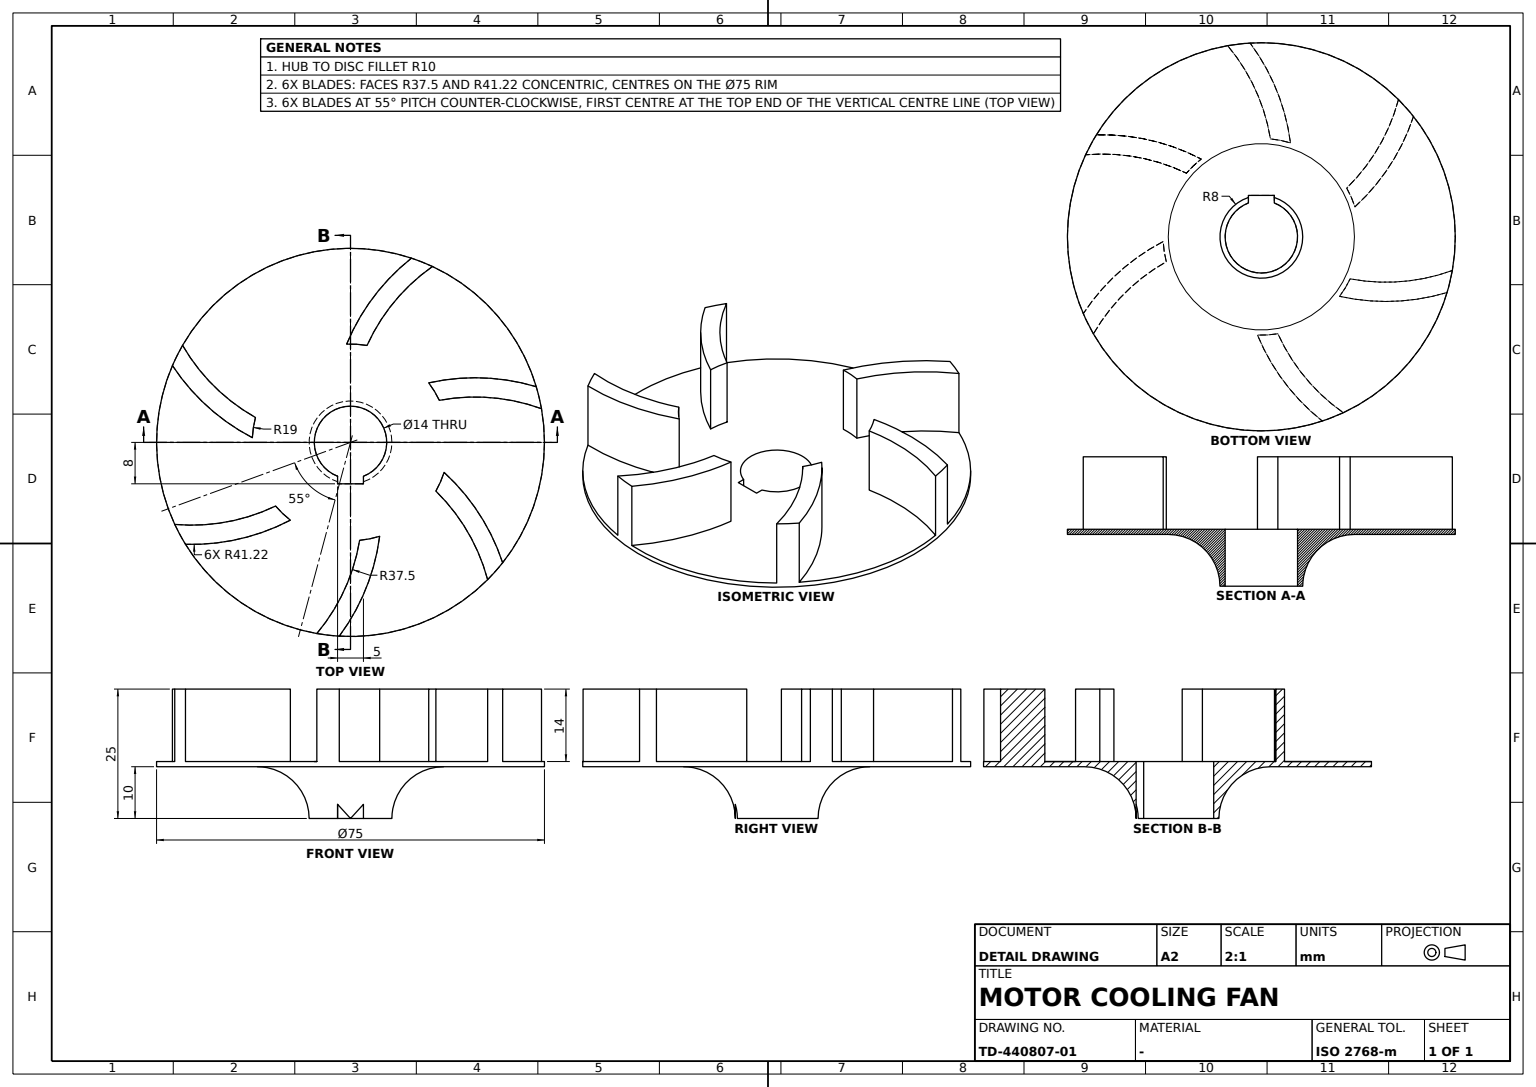
ISO-10303-21;
HEADER;
FILE_DESCRIPTION((''),'2;1');
FILE_NAME('','',(''),(''),'','','');
FILE_SCHEMA(('AUTOMOTIVE_DESIGN'));
ENDSEC;
DATA;
#1=APPLICATION_CONTEXT('');
#2=PRODUCT_CONTEXT('',#1,'mechanical');
#3=PRODUCT('','','',(#2));
#4=PRODUCT_DEFINITION_FORMATION('','',#3);
#5=PRODUCT_DEFINITION_CONTEXT('',#1,'design');
#6=PRODUCT_DEFINITION('','',#4,#5);
#7=PRODUCT_DEFINITION_SHAPE('','',#6);
#8=(LENGTH_UNIT()NAMED_UNIT(*)SI_UNIT(.MILLI.,.METRE.));
#9=(NAMED_UNIT(*)PLANE_ANGLE_UNIT()SI_UNIT($,.RADIAN.));
#10=(NAMED_UNIT(*)SI_UNIT($,.STERADIAN.)SOLID_ANGLE_UNIT());
#11=UNCERTAINTY_MEASURE_WITH_UNIT(LENGTH_MEASURE(0.005),#8,'distance_accuracy_value','');
#12=(GEOMETRIC_REPRESENTATION_CONTEXT(3)GLOBAL_UNCERTAINTY_ASSIGNED_CONTEXT((#11))GLOBAL_UNIT_ASSIGNED_CONTEXT((#8,#9,#10))REPRESENTATION_CONTEXT('',''));
#13=CARTESIAN_POINT('',(5.636932,-18.144558,1.));
#14=VERTEX_POINT('',#13);
#15=CARTESIAN_POINT('',(5.636932,-18.144558,15.));
#16=VERTEX_POINT('',#15);
#17=DIRECTION('',(0.,0.,1.));
#18=VECTOR('',#17,1000.);
#19=LINE('',#13,#18);
#20=EDGE_CURVE('',#14,#16,#19,.T.);
#21=ORIENTED_EDGE('',*,*,#20,.T.);
#22=CARTESIAN_POINT('',(-2.172274,-37.43703,15.));
#23=VERTEX_POINT('',#22);
#24=CARTESIAN_POINT('',(-35.238473,-12.825755,15.));
#25=DIRECTION('',(1.,0.,0.));
#26=AXIS2_PLACEMENT_3D('',#24,#17,#25);
#27=CIRCLE('',#26,41.22);
#28=EDGE_CURVE('',#23,#16,#27,.T.);
#29=ORIENTED_EDGE('',*,*,#28,.F.);
#30=CARTESIAN_POINT('',(-2.172274,-37.43703,1.));
#31=VERTEX_POINT('',#30);
#32=LINE('',#30,#18);
#33=EDGE_CURVE('',#31,#23,#32,.T.);
#34=ORIENTED_EDGE('',*,*,#33,.F.);
#35=CARTESIAN_POINT('',(-35.238473,-12.825755,1.));
#36=AXIS2_PLACEMENT_3D('',#35,#17,#25);
#37=CIRCLE('',#36,41.22);
#38=EDGE_CURVE('',#31,#14,#37,.T.);
#39=ORIENTED_EDGE('',*,*,#38,.T.);
#40=EDGE_LOOP('',(#21,#29,#34,#39));
#41=FACE_BOUND('',#40,.T.);
#42=CARTESIAN_POINT('',(-35.238473,-12.825755,8.));
#43=DIRECTION('',(-0.342020143,0.939692621,0.));
#44=AXIS2_PLACEMENT_3D('',#42,#17,#43);
#45=CYLINDRICAL_SURFACE('',#44,41.22);
#46=ADVANCED_FACE('',(#41),#45,.T.);
#47=CARTESIAN_POINT('',(2.5,-6.538348,1.));
#48=VERTEX_POINT('',#47);
#49=CARTESIAN_POINT('',(2.5,-8.,1.));
#50=VERTEX_POINT('',#49);
#51=CARTESIAN_POINT('',(2.5,0.,1.));
#52=DIRECTION('',(0.,-1.,0.));
#53=VECTOR('',#52,1000.);
#54=LINE('',#51,#53);
#55=EDGE_CURVE('',#48,#50,#54,.T.);
#56=ORIENTED_EDGE('',*,*,#55,.F.);
#57=CARTESIAN_POINT('',(2.5,-6.538348,-10.));
#58=VERTEX_POINT('',#57);
#59=DIRECTION('',(0.,0.,-1.));
#60=VECTOR('',#59,1000.);
#61=LINE('',#57,#60);
#62=EDGE_CURVE('',#58,#48,#61,.F.);
#63=ORIENTED_EDGE('',*,*,#62,.F.);
#64=CARTESIAN_POINT('',(2.5,-7.599342,-10.));
#65=VERTEX_POINT('',#64);
#66=LINE('',#57,#53);
#67=EDGE_CURVE('',#58,#65,#66,.T.);
#68=ORIENTED_EDGE('',*,*,#67,.T.);
#69=CARTESIAN_POINT('',(2.5,-8.,-7.264131));
#70=VERTEX_POINT('',#69);
#71=CARTESIAN_POINT('',(2.5,-7.734013,-8.156693));
#72=CARTESIAN_POINT('',(2.5,-7.599342,-9.068485));
#73=B_SPLINE_CURVE_WITH_KNOTS('',3,(#69,#71,#72,#64),.UNSPECIFIED.,.F.,.F.,(4,4),(0.,0.002765051),.UNSPECIFIED.);
#74=EDGE_CURVE('',#70,#65,#73,.T.);
#75=ORIENTED_EDGE('',*,*,#74,.F.);
#76=CARTESIAN_POINT('',(2.5,-8.,-10.));
#77=LINE('',#76,#60);
#78=EDGE_CURVE('',#50,#70,#77,.T.);
#79=ORIENTED_EDGE('',*,*,#78,.F.);
#80=EDGE_LOOP('',(#56,#63,#68,#75,#79));
#81=FACE_BOUND('',#80,.T.);
#82=DIRECTION('',(-1.,0.,0.));
#83=AXIS2_PLACEMENT_3D('',#57,#82,#52);
#84=PLANE('',#83);
#85=ADVANCED_FACE('',(#81),#84,.T.);
#86=CARTESIAN_POINT('',(3.193077,18.729769,1.));
#87=VERTEX_POINT('',#86);
#88=CARTESIAN_POINT('',(3.193077,18.729769,15.));
#89=VERTEX_POINT('',#88);
#90=LINE('',#86,#18);
#91=EDGE_CURVE('',#87,#89,#90,.T.);
#92=ORIENTED_EDGE('',*,*,#91,.F.);
#93=CARTESIAN_POINT('',(15.848185,33.986542,1.));
#94=VERTEX_POINT('',#93);
#95=CARTESIAN_POINT('',(37.357301,3.26834,1.));
#96=AXIS2_PLACEMENT_3D('',#95,#17,#25);
#97=CIRCLE('',#96,37.5);
#98=EDGE_CURVE('',#94,#87,#97,.T.);
#99=ORIENTED_EDGE('',*,*,#98,.F.);
#100=CARTESIAN_POINT('',(15.848185,33.986542,15.));
#101=VERTEX_POINT('',#100);
#102=LINE('',#93,#18);
#103=EDGE_CURVE('',#94,#101,#102,.T.);
#104=ORIENTED_EDGE('',*,*,#103,.T.);
#105=CARTESIAN_POINT('',(37.357301,3.26834,15.));
#106=AXIS2_PLACEMENT_3D('',#105,#17,#25);
#107=CIRCLE('',#106,37.5);
#108=EDGE_CURVE('',#101,#89,#107,.T.);
#109=ORIENTED_EDGE('',*,*,#108,.T.);
#110=EDGE_LOOP('',(#92,#99,#104,#109));
#111=FACE_BOUND('',#110,.T.);
#112=CARTESIAN_POINT('',(37.357301,3.26834,8.));
#113=DIRECTION('',(0.087155743,-0.996194698,0.));
#114=AXIS2_PLACEMENT_3D('',#112,#17,#113);
#115=CYLINDRICAL_SURFACE('',#114,37.5);
#116=ADVANCED_FACE('',(#111),#115,.F.);
#117=CARTESIAN_POINT('',(-32.475953,18.75,1.));
#118=VERTEX_POINT('',#117);
#119=CARTESIAN_POINT('',(-32.475953,18.75,15.));
#120=VERTEX_POINT('',#119);
#121=LINE('',#117,#18);
#122=EDGE_CURVE('',#118,#120,#121,.T.);
#123=ORIENTED_EDGE('',*,*,#122,.T.);
#124=CARTESIAN_POINT('',(-18.380202,4.813333,15.));
#125=VERTEX_POINT('',#124);
#126=CARTESIAN_POINT('',(0.,37.5,15.));
#127=AXIS2_PLACEMENT_3D('',#126,#17,#25);
#128=CIRCLE('',#127,37.5);
#129=EDGE_CURVE('',#120,#125,#128,.T.);
#130=ORIENTED_EDGE('',*,*,#129,.T.);
#131=CARTESIAN_POINT('',(-18.380202,4.813333,1.));
#132=VERTEX_POINT('',#131);
#133=LINE('',#131,#18);
#134=EDGE_CURVE('',#132,#125,#133,.T.);
#135=ORIENTED_EDGE('',*,*,#134,.F.);
#136=CARTESIAN_POINT('',(0.,37.5,1.));
#137=AXIS2_PLACEMENT_3D('',#136,#17,#25);
#138=CIRCLE('',#137,37.5);
#139=EDGE_CURVE('',#118,#132,#138,.T.);
#140=ORIENTED_EDGE('',*,*,#139,.F.);
#141=EDGE_LOOP('',(#123,#130,#135,#140));
#142=FACE_BOUND('',#141,.T.);
#143=CARTESIAN_POINT('',(0.,37.5,8.));
#144=AXIS2_PLACEMENT_3D('',#143,#17,#25);
#145=CYLINDRICAL_SURFACE('',#144,37.5);
#146=ADVANCED_FACE('',(#142),#145,.F.);
#147=ORIENTED_EDGE('',*,*,#67,.F.);
#148=CARTESIAN_POINT('',(-2.5,-6.538348,-10.));
#149=VERTEX_POINT('',#148);
#150=CARTESIAN_POINT('',(0.,0.,-10.));
#151=AXIS2_PLACEMENT_3D('',#150,#59,#82);
#152=CIRCLE('',#151,7.);
#153=EDGE_CURVE('',#149,#58,#152,.T.);
#154=ORIENTED_EDGE('',*,*,#153,.F.);
#155=CARTESIAN_POINT('',(-2.5,-7.599342,-10.));
#156=VERTEX_POINT('',#155);
#157=LINE('',#148,#53);
#158=EDGE_CURVE('',#149,#156,#157,.T.);
#159=ORIENTED_EDGE('',*,*,#158,.T.);
#160=AXIS2_PLACEMENT_3D('',#150,#17,#25);
#161=CIRCLE('',#160,8.);
#162=EDGE_CURVE('',#156,#65,#161,.F.);
#163=ORIENTED_EDGE('',*,*,#162,.T.);
#164=EDGE_LOOP('',(#147,#154,#159,#163));
#165=FACE_BOUND('',#164,.T.);
#166=AXIS2_PLACEMENT_3D('',#150,#59,#25);
#167=PLANE('',#166);
#168=ADVANCED_FACE('',(#165),#167,.T.);
#169=CARTESIAN_POINT('',(-2.5,-6.538348,1.));
#170=VERTEX_POINT('',#169);
#171=CARTESIAN_POINT('',(-2.5,-8.,1.));
#172=VERTEX_POINT('',#171);
#173=CARTESIAN_POINT('',(-2.5,0.,1.));
#174=LINE('',#173,#53);
#175=EDGE_CURVE('',#170,#172,#174,.T.);
#176=ORIENTED_EDGE('',*,*,#175,.T.);
#177=CARTESIAN_POINT('',(-2.5,-8.,-7.26413));
#178=VERTEX_POINT('',#177);
#179=CARTESIAN_POINT('',(-2.5,-8.,-10.));
#180=LINE('',#179,#60);
#181=EDGE_CURVE('',#172,#178,#180,.T.);
#182=ORIENTED_EDGE('',*,*,#181,.T.);
#183=CARTESIAN_POINT('',(-2.5,-7.599342,-9.068485));
#184=CARTESIAN_POINT('',(-2.5,-7.734013,-8.156692));
#185=B_SPLINE_CURVE_WITH_KNOTS('',3,(#155,#183,#184,#177),.UNSPECIFIED.,.F.,.F.,(4,4),(0.,0.002765051),.UNSPECIFIED.);
#186=EDGE_CURVE('',#156,#178,#185,.T.);
#187=ORIENTED_EDGE('',*,*,#186,.F.);
#188=ORIENTED_EDGE('',*,*,#158,.F.);
#189=LINE('',#148,#60);
#190=EDGE_CURVE('',#149,#170,#189,.F.);
#191=ORIENTED_EDGE('',*,*,#190,.T.);
#192=EDGE_LOOP('',(#176,#182,#187,#188,#191));
#193=FACE_BOUND('',#192,.T.);
#194=AXIS2_PLACEMENT_3D('',#148,#82,#52);
#195=PLANE('',#194);
#196=ADVANCED_FACE('',(#193),#195,.F.);
#197=CARTESIAN_POINT('',(36.930291,6.511807,15.));
#198=VERTEX_POINT('',#197);
#199=CARTESIAN_POINT('',(35.922262,10.762949,15.));
#200=VERTEX_POINT('',#199);
#201=CARTESIAN_POINT('',(0.,0.,15.));
#202=AXIS2_PLACEMENT_3D('',#201,#17,#25);
#203=CIRCLE('',#202,37.5);
#204=EDGE_CURVE('',#198,#200,#203,.T.);
#205=ORIENTED_EDGE('',*,*,#204,.T.);
#206=CARTESIAN_POINT('',(15.122363,11.502788,15.));
#207=VERTEX_POINT('',#206);
#208=CARTESIAN_POINT('',(24.104535,-28.726667,15.));
#209=AXIS2_PLACEMENT_3D('',#208,#17,#25);
#210=CIRCLE('',#209,41.22);
#211=EDGE_CURVE('',#200,#207,#210,.T.);
#212=ORIENTED_EDGE('',*,*,#211,.T.);
#213=CARTESIAN_POINT('',(17.174003,8.127339,15.));
#214=VERTEX_POINT('',#213);
#215=CIRCLE('',#202,19.);
#216=EDGE_CURVE('',#214,#207,#215,.T.);
#217=ORIENTED_EDGE('',*,*,#216,.F.);
#218=CIRCLE('',#209,37.5);
#219=EDGE_CURVE('',#198,#214,#218,.T.);
#220=ORIENTED_EDGE('',*,*,#219,.F.);
#221=EDGE_LOOP('',(#205,#212,#217,#220));
#222=FACE_BOUND('',#221,.T.);
#223=PLANE('',#202);
#224=ADVANCED_FACE('',(#222),#223,.T.);
#225=CARTESIAN_POINT('',(26.516504,-26.516504,1.));
#226=VERTEX_POINT('',#225);
#227=CARTESIAN_POINT('',(16.508129,-9.406469,1.));
#228=VERTEX_POINT('',#227);
#229=CARTESIAN_POINT('',(-9.705714,-36.222218,1.));
#230=AXIS2_PLACEMENT_3D('',#229,#17,#25);
#231=CIRCLE('',#230,37.5);
#232=EDGE_CURVE('',#226,#228,#231,.T.);
#233=ORIENTED_EDGE('',*,*,#232,.T.);
#234=CARTESIAN_POINT('',(18.096363,-5.789787,1.));
#235=VERTEX_POINT('',#234);
#236=CARTESIAN_POINT('',(0.,0.,1.));
#237=AXIS2_PLACEMENT_3D('',#236,#17,#25);
#238=CIRCLE('',#237,19.);
#239=EDGE_CURVE('',#228,#235,#238,.T.);
#240=ORIENTED_EDGE('',*,*,#239,.T.);
#241=CARTESIAN_POINT('',(29.420655,-23.252421,1.));
#242=VERTEX_POINT('',#241);
#243=CIRCLE('',#230,41.22);
#244=EDGE_CURVE('',#242,#235,#243,.T.);
#245=ORIENTED_EDGE('',*,*,#244,.F.);
#246=CARTESIAN_POINT('',(36.930291,6.511807,1.));
#247=VERTEX_POINT('',#246);
#248=CIRCLE('',#237,37.5);
#249=EDGE_CURVE('',#242,#247,#248,.T.);
#250=ORIENTED_EDGE('',*,*,#249,.T.);
#251=CARTESIAN_POINT('',(17.174003,8.127339,1.));
#252=VERTEX_POINT('',#251);
#253=CARTESIAN_POINT('',(24.104535,-28.726667,1.));
#254=AXIS2_PLACEMENT_3D('',#253,#17,#25);
#255=CIRCLE('',#254,37.5);
#256=EDGE_CURVE('',#247,#252,#255,.T.);
#257=ORIENTED_EDGE('',*,*,#256,.T.);
#258=CARTESIAN_POINT('',(15.122363,11.502788,1.));
#259=VERTEX_POINT('',#258);
#260=EDGE_CURVE('',#252,#259,#238,.T.);
#261=ORIENTED_EDGE('',*,*,#260,.T.);
#262=CARTESIAN_POINT('',(35.922262,10.762949,1.));
#263=VERTEX_POINT('',#262);
#264=CIRCLE('',#254,41.22);
#265=EDGE_CURVE('',#263,#259,#264,.T.);
#266=ORIENTED_EDGE('',*,*,#265,.F.);
#267=EDGE_CURVE('',#263,#94,#248,.T.);
#268=ORIENTED_EDGE('',*,*,#267,.T.);
#269=ORIENTED_EDGE('',*,*,#98,.T.);
#270=CARTESIAN_POINT('',(-0.748701,18.985243,1.));
#271=VERTEX_POINT('',#270);
#272=EDGE_CURVE('',#87,#271,#238,.T.);
#273=ORIENTED_EDGE('',*,*,#272,.T.);
#274=CARTESIAN_POINT('',(11.787672,35.599168,1.));
#275=VERTEX_POINT('',#274);
#276=CIRCLE('',#96,41.22);
#277=EDGE_CURVE('',#275,#271,#276,.T.);
#278=ORIENTED_EDGE('',*,*,#277,.F.);
#279=EDGE_CURVE('',#275,#118,#248,.T.);
#280=ORIENTED_EDGE('',*,*,#279,.T.);
#281=ORIENTED_EDGE('',*,*,#139,.T.);
#282=CARTESIAN_POINT('',(-18.978252,0.908821,1.));
#283=VERTEX_POINT('',#282);
#284=EDGE_CURVE('',#132,#283,#238,.T.);
#285=ORIENTED_EDGE('',*,*,#284,.T.);
#286=CARTESIAN_POINT('',(-34.43634,14.845488,1.));
#287=VERTEX_POINT('',#286);
#288=CIRCLE('',#137,41.22);
#289=EDGE_CURVE('',#287,#283,#288,.T.);
#290=ORIENTED_EDGE('',*,*,#289,.F.);
#291=CARTESIAN_POINT('',(-33.986542,-15.848185,1.));
#292=VERTEX_POINT('',#291);
#293=EDGE_CURVE('',#287,#292,#248,.T.);
#294=ORIENTED_EDGE('',*,*,#293,.T.);
#295=CARTESIAN_POINT('',(-14.485303,-12.295365,1.));
#296=VERTEX_POINT('',#295);
#297=CARTESIAN_POINT('',(-30.718202,21.509116,1.));
#298=AXIS2_PLACEMENT_3D('',#297,#17,#25);
#299=CIRCLE('',#298,37.5);
#300=EDGE_CURVE('',#292,#296,#299,.T.);
#301=ORIENTED_EDGE('',*,*,#300,.T.);
#302=CARTESIAN_POINT('',(-11.629941,-15.024795,1.));
#303=VERTEX_POINT('',#302);
#304=EDGE_CURVE('',#296,#303,#238,.T.);
#305=ORIENTED_EDGE('',*,*,#304,.T.);
#306=CARTESIAN_POINT('',(-31.912585,-19.693576,1.));
#307=VERTEX_POINT('',#306);
#308=CIRCLE('',#298,41.22);
#309=EDGE_CURVE('',#307,#303,#308,.T.);
#310=ORIENTED_EDGE('',*,*,#309,.F.);
#311=CARTESIAN_POINT('',(-6.511807,-36.930291,1.));
#312=VERTEX_POINT('',#311);
#313=EDGE_CURVE('',#307,#312,#248,.T.);
#314=ORIENTED_EDGE('',*,*,#313,.T.);
#315=CARTESIAN_POINT('',(1.763345,-18.917997,1.));
#316=VERTEX_POINT('',#315);
#317=CIRCLE('',#36,37.5);
#318=EDGE_CURVE('',#312,#316,#317,.T.);
#319=ORIENTED_EDGE('',*,*,#318,.T.);
#320=EDGE_CURVE('',#316,#14,#238,.T.);
#321=ORIENTED_EDGE('',*,*,#320,.T.);
#322=ORIENTED_EDGE('',*,*,#38,.F.);
#323=EDGE_CURVE('',#31,#226,#248,.T.);
#324=ORIENTED_EDGE('',*,*,#323,.T.);
#325=EDGE_LOOP('',(#233,#240,#245,#250,#257,#261,#266,#268,#269,#273,#278,#280,#281,#285,#290,#294,#301,#305,#310,#314,#319,#321,#322,#324));
#326=FACE_BOUND('',#325,.T.);
#327=CARTESIAN_POINT('',(0.,-8.,1.));
#328=VECTOR('',#25,1000.);
#329=LINE('',#327,#328);
#330=EDGE_CURVE('',#172,#50,#329,.T.);
#331=ORIENTED_EDGE('',*,*,#330,.F.);
#332=ORIENTED_EDGE('',*,*,#175,.F.);
#333=CIRCLE('',#237,7.);
#334=EDGE_CURVE('',#48,#170,#333,.T.);
#335=ORIENTED_EDGE('',*,*,#334,.F.);
#336=ORIENTED_EDGE('',*,*,#55,.T.);
#337=EDGE_LOOP('',(#331,#332,#335,#336));
#338=FACE_BOUND('',#337,.T.);
#339=PLANE('',#237);
#340=ADVANCED_FACE('',(#326,#338),#339,.T.);
#341=CARTESIAN_POINT('',(-34.43634,14.845488,15.));
#342=VERTEX_POINT('',#341);
#343=EDGE_CURVE('',#120,#342,#203,.T.);
#344=ORIENTED_EDGE('',*,*,#343,.T.);
#345=CARTESIAN_POINT('',(-18.978252,0.908821,15.));
#346=VERTEX_POINT('',#345);
#347=CIRCLE('',#127,41.22);
#348=EDGE_CURVE('',#342,#346,#347,.T.);
#349=ORIENTED_EDGE('',*,*,#348,.T.);
#350=EDGE_CURVE('',#125,#346,#215,.T.);
#351=ORIENTED_EDGE('',*,*,#350,.F.);
#352=ORIENTED_EDGE('',*,*,#129,.F.);
#353=EDGE_LOOP('',(#344,#349,#351,#352));
#354=FACE_BOUND('',#353,.T.);
#355=ADVANCED_FACE('',(#354),#223,.T.);
#356=CARTESIAN_POINT('',(37.5,0.,0.));
#357=VERTEX_POINT('',#356);
#358=CARTESIAN_POINT('',(0.,0.,0.));
#359=AXIS2_PLACEMENT_3D('',#358,#17,#25);
#360=CIRCLE('',#359,37.5);
#361=EDGE_CURVE('',#357,#357,#360,.T.);
#362=ORIENTED_EDGE('',*,*,#361,.F.);
#363=EDGE_LOOP('',(#362));
#364=FACE_BOUND('',#363,.T.);
#365=CARTESIAN_POINT('',(18.,0.,0.));
#366=VERTEX_POINT('',#365);
#367=CIRCLE('',#359,18.);
#368=EDGE_CURVE('',#366,#366,#367,.T.);
#369=ORIENTED_EDGE('',*,*,#368,.T.);
#370=EDGE_LOOP('',(#369));
#371=FACE_BOUND('',#370,.T.);
#372=PLANE('',#359);
#373=ADVANCED_FACE('',(#364,#371),#372,.F.);
#374=ORIENTED_EDGE('',*,*,#91,.T.);
#375=CARTESIAN_POINT('',(-0.748701,18.985243,15.));
#376=VERTEX_POINT('',#375);
#377=EDGE_CURVE('',#89,#376,#215,.T.);
#378=ORIENTED_EDGE('',*,*,#377,.T.);
#379=LINE('',#270,#18);
#380=EDGE_CURVE('',#271,#376,#379,.T.);
#381=ORIENTED_EDGE('',*,*,#380,.F.);
#382=ORIENTED_EDGE('',*,*,#272,.F.);
#383=EDGE_LOOP('',(#374,#378,#381,#382));
#384=FACE_BOUND('',#383,.T.);
#385=CARTESIAN_POINT('',(0.,0.,8.));
#386=DIRECTION('',(0.573576436,0.819152044,0.));
#387=AXIS2_PLACEMENT_3D('',#385,#17,#386);
#388=CYLINDRICAL_SURFACE('',#387,19.);
#389=ADVANCED_FACE('',(#384),#388,.F.);
#390=ORIENTED_EDGE('',*,*,#350,.T.);
#391=LINE('',#282,#18);
#392=EDGE_CURVE('',#283,#346,#391,.T.);
#393=ORIENTED_EDGE('',*,*,#392,.F.);
#394=ORIENTED_EDGE('',*,*,#284,.F.);
#395=ORIENTED_EDGE('',*,*,#134,.T.);
#396=EDGE_LOOP('',(#390,#393,#394,#395));
#397=FACE_BOUND('',#396,.T.);
#398=ADVANCED_FACE('',(#397),#388,.F.);
#399=ORIENTED_EDGE('',*,*,#318,.F.);
#400=CARTESIAN_POINT('',(-6.511807,-36.930291,15.));
#401=VERTEX_POINT('',#400);
#402=LINE('',#311,#18);
#403=EDGE_CURVE('',#312,#401,#402,.T.);
#404=ORIENTED_EDGE('',*,*,#403,.T.);
#405=CARTESIAN_POINT('',(1.763345,-18.917997,15.));
#406=VERTEX_POINT('',#405);
#407=CIRCLE('',#26,37.5);
#408=EDGE_CURVE('',#401,#406,#407,.T.);
#409=ORIENTED_EDGE('',*,*,#408,.T.);
#410=LINE('',#315,#18);
#411=EDGE_CURVE('',#316,#406,#410,.T.);
#412=ORIENTED_EDGE('',*,*,#411,.F.);
#413=EDGE_LOOP('',(#399,#404,#409,#412));
#414=FACE_BOUND('',#413,.T.);
#415=CYLINDRICAL_SURFACE('',#44,37.5);
#416=ADVANCED_FACE('',(#414),#415,.F.);
#417=CARTESIAN_POINT('',(0.,-8.,-10.));
#418=VERTEX_POINT('',#417);
#419=CARTESIAN_POINT('',(-1.647259,-8.,-8.158351));
#420=CARTESIAN_POINT('',(-0.823572,-8.,-9.079219));
#421=B_SPLINE_CURVE_WITH_KNOTS('',3,(#177,#419,#420,#417),.UNSPECIFIED.,.F.,.F.,(4,4),(0.,0.003706075),.UNSPECIFIED.);
#422=EDGE_CURVE('',#178,#418,#421,.T.);
#423=ORIENTED_EDGE('',*,*,#422,.T.);
#424=CARTESIAN_POINT('',(2.5,-8.,-7.26413));
#425=CARTESIAN_POINT('',(1.647259,-8.,-8.158351));
#426=CARTESIAN_POINT('',(0.823572,-8.,-9.079219));
#427=B_SPLINE_CURVE_WITH_KNOTS('',3,(#424,#425,#426,#417),.UNSPECIFIED.,.F.,.F.,(4,4),(0.,0.003706075),.UNSPECIFIED.);
#428=EDGE_CURVE('',#418,#70,#427,.F.);
#429=ORIENTED_EDGE('',*,*,#428,.T.);
#430=ORIENTED_EDGE('',*,*,#74,.T.);
#431=ORIENTED_EDGE('',*,*,#162,.F.);
#432=ORIENTED_EDGE('',*,*,#186,.T.);
#433=EDGE_LOOP('',(#423,#429,#430,#431,#432));
#434=FACE_BOUND('',#433,.T.);
#435=ORIENTED_EDGE('',*,*,#368,.F.);
#436=EDGE_LOOP('',(#435));
#437=FACE_BOUND('',#436,.T.);
#438=DIRECTION('',(0.866025404,-0.5,0.));
#439=AXIS2_PLACEMENT_3D('',#150,#17,#438);
#440=TOROIDAL_SURFACE('',#439,18.,10.);
#441=ADVANCED_FACE('',(#434,#437),#440,.F.);
#442=ORIENTED_EDGE('',*,*,#256,.F.);
#443=LINE('',#246,#18);
#444=EDGE_CURVE('',#247,#198,#443,.T.);
#445=ORIENTED_EDGE('',*,*,#444,.T.);
#446=ORIENTED_EDGE('',*,*,#219,.T.);
#447=LINE('',#251,#18);
#448=EDGE_CURVE('',#252,#214,#447,.T.);
#449=ORIENTED_EDGE('',*,*,#448,.F.);
#450=EDGE_LOOP('',(#442,#445,#446,#449));
#451=FACE_BOUND('',#450,.T.);
#452=CARTESIAN_POINT('',(24.104535,-28.726667,8.));
#453=DIRECTION('',(-0.766044443,-0.64278761,0.));
#454=AXIS2_PLACEMENT_3D('',#452,#17,#453);
#455=CYLINDRICAL_SURFACE('',#454,37.5);
#456=ADVANCED_FACE('',(#451),#455,.F.);
#457=ORIENTED_EDGE('',*,*,#428,.F.);
#458=ORIENTED_EDGE('',*,*,#422,.F.);
#459=ORIENTED_EDGE('',*,*,#181,.F.);
#460=ORIENTED_EDGE('',*,*,#330,.T.);
#461=ORIENTED_EDGE('',*,*,#78,.T.);
#462=EDGE_LOOP('',(#457,#458,#459,#460,#461));
#463=FACE_BOUND('',#462,.T.);
#464=AXIS2_PLACEMENT_3D('',#179,#52,#25);
#465=PLANE('',#464);
#466=ADVANCED_FACE('',(#463),#465,.F.);
#467=ORIENTED_EDGE('',*,*,#380,.T.);
#468=CARTESIAN_POINT('',(11.787672,35.599168,15.));
#469=VERTEX_POINT('',#468);
#470=CIRCLE('',#106,41.22);
#471=EDGE_CURVE('',#469,#376,#470,.T.);
#472=ORIENTED_EDGE('',*,*,#471,.F.);
#473=LINE('',#274,#18);
#474=EDGE_CURVE('',#275,#469,#473,.T.);
#475=ORIENTED_EDGE('',*,*,#474,.F.);
#476=ORIENTED_EDGE('',*,*,#277,.T.);
#477=EDGE_LOOP('',(#467,#472,#475,#476));
#478=FACE_BOUND('',#477,.T.);
#479=CYLINDRICAL_SURFACE('',#114,41.22);
#480=ADVANCED_FACE('',(#478),#479,.T.);
#481=CARTESIAN_POINT('',(16.508129,-9.406469,15.));
#482=VERTEX_POINT('',#481);
#483=LINE('',#227,#18);
#484=EDGE_CURVE('',#228,#482,#483,.T.);
#485=ORIENTED_EDGE('',*,*,#484,.T.);
#486=CARTESIAN_POINT('',(18.096363,-5.789787,15.));
#487=VERTEX_POINT('',#486);
#488=EDGE_CURVE('',#482,#487,#215,.T.);
#489=ORIENTED_EDGE('',*,*,#488,.T.);
#490=LINE('',#234,#18);
#491=EDGE_CURVE('',#235,#487,#490,.T.);
#492=ORIENTED_EDGE('',*,*,#491,.F.);
#493=ORIENTED_EDGE('',*,*,#239,.F.);
#494=EDGE_LOOP('',(#485,#489,#492,#493));
#495=FACE_BOUND('',#494,.T.);
#496=ADVANCED_FACE('',(#495),#388,.F.);
#497=ORIENTED_EDGE('',*,*,#265,.T.);
#498=LINE('',#258,#18);
#499=EDGE_CURVE('',#259,#207,#498,.T.);
#500=ORIENTED_EDGE('',*,*,#499,.T.);
#501=ORIENTED_EDGE('',*,*,#211,.F.);
#502=LINE('',#262,#18);
#503=EDGE_CURVE('',#263,#200,#502,.T.);
#504=ORIENTED_EDGE('',*,*,#503,.F.);
#505=EDGE_LOOP('',(#497,#500,#501,#504));
#506=FACE_BOUND('',#505,.T.);
#507=CYLINDRICAL_SURFACE('',#454,41.22);
#508=ADVANCED_FACE('',(#506),#507,.T.);
#509=EDGE_CURVE('',#401,#23,#203,.T.);
#510=ORIENTED_EDGE('',*,*,#509,.T.);
#511=ORIENTED_EDGE('',*,*,#28,.T.);
#512=EDGE_CURVE('',#406,#16,#215,.T.);
#513=ORIENTED_EDGE('',*,*,#512,.F.);
#514=ORIENTED_EDGE('',*,*,#408,.F.);
#515=EDGE_LOOP('',(#510,#511,#513,#514));
#516=FACE_BOUND('',#515,.T.);
#517=ADVANCED_FACE('',(#516),#223,.T.);
#518=ORIENTED_EDGE('',*,*,#448,.T.);
#519=ORIENTED_EDGE('',*,*,#216,.T.);
#520=ORIENTED_EDGE('',*,*,#499,.F.);
#521=ORIENTED_EDGE('',*,*,#260,.F.);
#522=EDGE_LOOP('',(#518,#519,#520,#521));
#523=FACE_BOUND('',#522,.T.);
#524=ADVANCED_FACE('',(#523),#388,.F.);
#525=CARTESIAN_POINT('',(-31.912585,-19.693576,15.));
#526=VERTEX_POINT('',#525);
#527=CARTESIAN_POINT('',(-11.629941,-15.024795,15.));
#528=VERTEX_POINT('',#527);
#529=CARTESIAN_POINT('',(-30.718202,21.509116,15.));
#530=AXIS2_PLACEMENT_3D('',#529,#17,#25);
#531=CIRCLE('',#530,41.22);
#532=EDGE_CURVE('',#526,#528,#531,.T.);
#533=ORIENTED_EDGE('',*,*,#532,.F.);
#534=LINE('',#306,#18);
#535=EDGE_CURVE('',#307,#526,#534,.T.);
#536=ORIENTED_EDGE('',*,*,#535,.F.);
#537=ORIENTED_EDGE('',*,*,#309,.T.);
#538=LINE('',#302,#18);
#539=EDGE_CURVE('',#303,#528,#538,.T.);
#540=ORIENTED_EDGE('',*,*,#539,.T.);
#541=EDGE_LOOP('',(#533,#536,#537,#540));
#542=FACE_BOUND('',#541,.T.);
#543=CARTESIAN_POINT('',(-30.718202,21.509116,8.));
#544=AXIS2_PLACEMENT_3D('',#543,#17,#386);
#545=CYLINDRICAL_SURFACE('',#544,41.22);
#546=ADVANCED_FACE('',(#542),#545,.T.);
#547=CARTESIAN_POINT('',(-33.986542,-15.848185,15.));
#548=VERTEX_POINT('',#547);
#549=EDGE_CURVE('',#548,#526,#203,.T.);
#550=ORIENTED_EDGE('',*,*,#549,.T.);
#551=ORIENTED_EDGE('',*,*,#532,.T.);
#552=CARTESIAN_POINT('',(-14.485303,-12.295365,15.));
#553=VERTEX_POINT('',#552);
#554=EDGE_CURVE('',#553,#528,#215,.T.);
#555=ORIENTED_EDGE('',*,*,#554,.F.);
#556=CIRCLE('',#530,37.5);
#557=EDGE_CURVE('',#548,#553,#556,.T.);
#558=ORIENTED_EDGE('',*,*,#557,.F.);
#559=EDGE_LOOP('',(#550,#551,#555,#558));
#560=FACE_BOUND('',#559,.T.);
#561=ADVANCED_FACE('',(#560),#223,.T.);
#562=ORIENTED_EDGE('',*,*,#539,.F.);
#563=ORIENTED_EDGE('',*,*,#304,.F.);
#564=LINE('',#295,#18);
#565=EDGE_CURVE('',#296,#553,#564,.T.);
#566=ORIENTED_EDGE('',*,*,#565,.T.);
#567=ORIENTED_EDGE('',*,*,#554,.T.);
#568=EDGE_LOOP('',(#562,#563,#566,#567));
#569=FACE_BOUND('',#568,.T.);
#570=ADVANCED_FACE('',(#569),#388,.F.);
#571=ORIENTED_EDGE('',*,*,#512,.T.);
#572=ORIENTED_EDGE('',*,*,#20,.F.);
#573=ORIENTED_EDGE('',*,*,#320,.F.);
#574=ORIENTED_EDGE('',*,*,#411,.T.);
#575=EDGE_LOOP('',(#571,#572,#573,#574));
#576=FACE_BOUND('',#575,.T.);
#577=ADVANCED_FACE('',(#576),#388,.F.);
#578=ORIENTED_EDGE('',*,*,#392,.T.);
#579=ORIENTED_EDGE('',*,*,#348,.F.);
#580=LINE('',#286,#18);
#581=EDGE_CURVE('',#287,#342,#580,.T.);
#582=ORIENTED_EDGE('',*,*,#581,.F.);
#583=ORIENTED_EDGE('',*,*,#289,.T.);
#584=EDGE_LOOP('',(#578,#579,#582,#583));
#585=FACE_BOUND('',#584,.T.);
#586=CYLINDRICAL_SURFACE('',#144,41.22);
#587=ADVANCED_FACE('',(#585),#586,.T.);
#588=ORIENTED_EDGE('',*,*,#491,.T.);
#589=CARTESIAN_POINT('',(29.420655,-23.252421,15.));
#590=VERTEX_POINT('',#589);
#591=CARTESIAN_POINT('',(-9.705714,-36.222218,15.));
#592=AXIS2_PLACEMENT_3D('',#591,#17,#25);
#593=CIRCLE('',#592,41.22);
#594=EDGE_CURVE('',#590,#487,#593,.T.);
#595=ORIENTED_EDGE('',*,*,#594,.F.);
#596=LINE('',#241,#18);
#597=EDGE_CURVE('',#242,#590,#596,.T.);
#598=ORIENTED_EDGE('',*,*,#597,.F.);
#599=ORIENTED_EDGE('',*,*,#244,.T.);
#600=EDGE_LOOP('',(#588,#595,#598,#599));
#601=FACE_BOUND('',#600,.T.);
#602=CARTESIAN_POINT('',(-9.705714,-36.222218,8.));
#603=DIRECTION('',(-0.965925826,0.258819045,0.));
#604=AXIS2_PLACEMENT_3D('',#602,#17,#603);
#605=CYLINDRICAL_SURFACE('',#604,41.22);
#606=ADVANCED_FACE('',(#601),#605,.T.);
#607=EDGE_CURVE('',#101,#469,#203,.T.);
#608=ORIENTED_EDGE('',*,*,#607,.T.);
#609=ORIENTED_EDGE('',*,*,#471,.T.);
#610=ORIENTED_EDGE('',*,*,#377,.F.);
#611=ORIENTED_EDGE('',*,*,#108,.F.);
#612=EDGE_LOOP('',(#608,#609,#610,#611));
#613=FACE_BOUND('',#612,.T.);
#614=ADVANCED_FACE('',(#613),#223,.T.);
#615=ORIENTED_EDGE('',*,*,#300,.F.);
#616=LINE('',#291,#18);
#617=EDGE_CURVE('',#292,#548,#616,.T.);
#618=ORIENTED_EDGE('',*,*,#617,.T.);
#619=ORIENTED_EDGE('',*,*,#557,.T.);
#620=ORIENTED_EDGE('',*,*,#565,.F.);
#621=EDGE_LOOP('',(#615,#618,#619,#620));
#622=FACE_BOUND('',#621,.T.);
#623=CYLINDRICAL_SURFACE('',#544,37.5);
#624=ADVANCED_FACE('',(#622),#623,.F.);
#625=ORIENTED_EDGE('',*,*,#190,.F.);
#626=ORIENTED_EDGE('',*,*,#153,.T.);
#627=ORIENTED_EDGE('',*,*,#62,.T.);
#628=ORIENTED_EDGE('',*,*,#334,.T.);
#629=EDGE_LOOP('',(#625,#626,#627,#628));
#630=FACE_BOUND('',#629,.T.);
#631=CARTESIAN_POINT('',(0.,0.,3.16));
#632=AXIS2_PLACEMENT_3D('',#631,#59,#25);
#633=CYLINDRICAL_SURFACE('',#632,7.);
#634=ADVANCED_FACE('',(#630),#633,.F.);
#635=CARTESIAN_POINT('',(26.516504,-26.516504,15.));
#636=VERTEX_POINT('',#635);
#637=CIRCLE('',#592,37.5);
#638=EDGE_CURVE('',#636,#482,#637,.T.);
#639=ORIENTED_EDGE('',*,*,#638,.T.);
#640=ORIENTED_EDGE('',*,*,#484,.F.);
#641=ORIENTED_EDGE('',*,*,#232,.F.);
#642=LINE('',#225,#18);
#643=EDGE_CURVE('',#226,#636,#642,.T.);
#644=ORIENTED_EDGE('',*,*,#643,.T.);
#645=EDGE_LOOP('',(#639,#640,#641,#644));
#646=FACE_BOUND('',#645,.T.);
#647=CYLINDRICAL_SURFACE('',#604,37.5);
#648=ADVANCED_FACE('',(#646),#647,.F.);
#649=ORIENTED_EDGE('',*,*,#594,.T.);
#650=ORIENTED_EDGE('',*,*,#488,.F.);
#651=ORIENTED_EDGE('',*,*,#638,.F.);
#652=EDGE_CURVE('',#636,#590,#203,.T.);
#653=ORIENTED_EDGE('',*,*,#652,.T.);
#654=EDGE_LOOP('',(#649,#650,#651,#653));
#655=FACE_BOUND('',#654,.T.);
#656=ADVANCED_FACE('',(#655),#223,.T.);
#657=ORIENTED_EDGE('',*,*,#361,.T.);
#658=EDGE_LOOP('',(#657));
#659=FACE_BOUND('',#658,.T.);
#660=ORIENTED_EDGE('',*,*,#33,.T.);
#661=ORIENTED_EDGE('',*,*,#509,.F.);
#662=ORIENTED_EDGE('',*,*,#403,.F.);
#663=ORIENTED_EDGE('',*,*,#313,.F.);
#664=ORIENTED_EDGE('',*,*,#535,.T.);
#665=ORIENTED_EDGE('',*,*,#549,.F.);
#666=ORIENTED_EDGE('',*,*,#617,.F.);
#667=ORIENTED_EDGE('',*,*,#293,.F.);
#668=ORIENTED_EDGE('',*,*,#581,.T.);
#669=ORIENTED_EDGE('',*,*,#343,.F.);
#670=ORIENTED_EDGE('',*,*,#122,.F.);
#671=ORIENTED_EDGE('',*,*,#279,.F.);
#672=ORIENTED_EDGE('',*,*,#474,.T.);
#673=ORIENTED_EDGE('',*,*,#607,.F.);
#674=ORIENTED_EDGE('',*,*,#103,.F.);
#675=ORIENTED_EDGE('',*,*,#267,.F.);
#676=ORIENTED_EDGE('',*,*,#503,.T.);
#677=ORIENTED_EDGE('',*,*,#204,.F.);
#678=ORIENTED_EDGE('',*,*,#444,.F.);
#679=ORIENTED_EDGE('',*,*,#249,.F.);
#680=ORIENTED_EDGE('',*,*,#597,.T.);
#681=ORIENTED_EDGE('',*,*,#652,.F.);
#682=ORIENTED_EDGE('',*,*,#643,.F.);
#683=ORIENTED_EDGE('',*,*,#323,.F.);
#684=EDGE_LOOP('',(#660,#661,#662,#663,#664,#665,#666,#667,#668,#669,#670,#671,#672,#673,#674,#675,#676,#677,#678,#679,#680,#681,#682,#683));
#685=FACE_BOUND('',#684,.T.);
#686=CARTESIAN_POINT('',(0.,0.,0.5));
#687=AXIS2_PLACEMENT_3D('',#686,#17,#25);
#688=CYLINDRICAL_SURFACE('',#687,37.5);
#689=ADVANCED_FACE('',(#659,#685),#688,.T.);
#690=CLOSED_SHELL('',(#46,#85,#116,#146,#168,#196,#224,#340,#355,#373,#389,#398,#416,#441,#456,#466,#480,#496,#508,#517,#524,#546,#561,#570,#577,#587,#606,#614,#624,#634,#648,#656,#689));
#691=MANIFOLD_SOLID_BREP('',#690);
#692=ADVANCED_BREP_SHAPE_REPRESENTATION('',(#691),#12);
#693=SHAPE_DEFINITION_REPRESENTATION(#7,#692);
ENDSEC;
END-ISO-10303-21;
